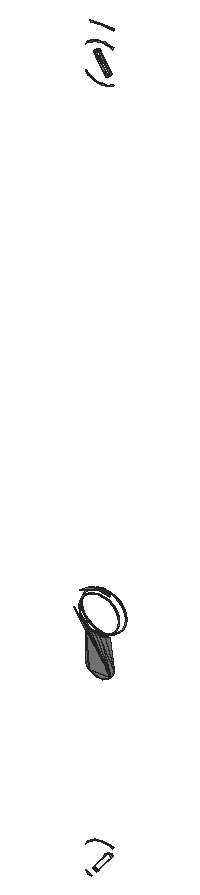
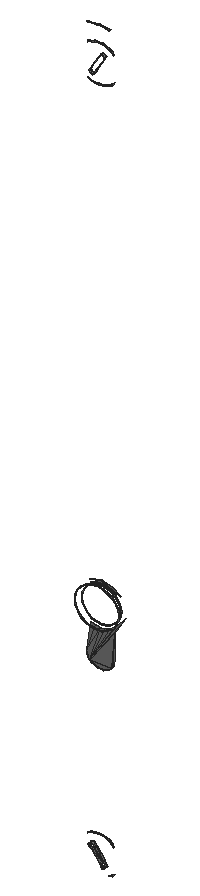
# SketchUp Ruby script. Lengths in inches.
U = 1.inch
M = Sketchup.active_model
def pt(a) = Geom::Point3d.new(a.map { |v| v * U })
def face(e, loops, mat)
  f = e.add_face(loops[0].map { |a| pt(a) })
  loops[1..].each { |l| e.add_face(l.map { |a| pt(a) }).erase! }
  f.material = f.back_material = mat if mat
  f
end
# faces: each face lists its corners as indices into pts; further lists are holes
def faces(e, pts, list, mat = nil) = list.each { |f| face(e, (f[0].is_a?(Array) ? f : [f]).map { |l| l.map { |i| pts[i] } }, mat) }
# xy, xz, yz: faces in a plane at the given z, y or x. An outline is a flat list of corners, or four numbers for a rectangle; further outlines are holes
def ring(l) = l.size == 4 ? [[l[0], l[1]], [l[2], l[1]], [l[2], l[3]], [l[0], l[3]]] : l.each_slice(2).to_a
def flat(e, list, mat, &to3) = list.each { |f| face(e, (f[0].is_a?(Array) ? f : [f]).map { |l| ring(l).map { |u, v| to3.(u, v) } }, mat) }
def xy(e, z, list, mat = nil) = flat(e, list, mat) { |x, y| [x, y, z] }
def xz(e, y, list, mat = nil) = flat(e, list, mat) { |x, z| [x, y, z] }
def yz(e, x, list, mat = nil) = flat(e, list, mat) { |y, z| [x, y, z] }
def lines(e, pts, list) = list.each { |a, b| e.add_line(pt(pts[a]), pt(pts[b])) }
# prism: a flat outline (further loops are holes) pulled along v
def prism(e, loops, v, mat = nil)
  f = face(e, loops, mat); d = Geom::Vector3d.new(v.map { |x| x * U })
  f.pushpull(f.normal.samedirection?(d) ? d.length : -d.length)
end
def box(e, o, s, mat = nil) = prism(e, [[o, [o[0] + s[0], o[1], o[2]], [o[0] + s[0], o[1] + s[1], o[2]], [o[0], o[1] + s[1], o[2]]]], [0, 0, s[2]], mat)
def at(x, y, z, deg = 0) = Geom::Transformation.translation(pt([x, y, z])) * Geom::Transformation.rotation(ORIGIN, Z_AXIS, deg.degrees)
def axes(o, x, y, z) = Geom::Transformation.new([*x, 0, *y, 0, *z, 0, *pt(o).to_a, 1])
def part(name) = M.definitions.add(name)
# library, detail: a bought-in or finely detailed component or shape, given as its bounding box
def library(name, o, s) = part(name).tap { |d| box(d.entities, o, s) }
def detail(e, o, s) = box(e.add_group.entities, o, s)
def put(e, d, t, mat = nil) = e.add_instance(d, t).tap { |i| i.material = mat if mat }
def group(e, t, mat = nil) = e.add_group.tap { |g| g.transformation = t; g.material = mat if mat }.entities
root = M.entities
M.materials.add("Material \#1").color = [140, 140, 140]
xz(root,529.302,[[1590.92,42.491,1590.851,42.499,1590.92,42.5],[1590.92,42.491,1590.92,42.5,1590.987,42.508],[1590.92,42.491,1590.987,42.508,1590.989,42.499],[1590.851,42.499,1590.786,42.523,1590.854,42.508],[1590.851,42.499,1590.854,42.508,1590.92,42.5],
  [1590.989,42.499,1590.987,42.508,1591.049,42.531],[1590.989,42.499,1591.049,42.531,1591.054,42.523],[1590.854,42.508,1590.786,42.523,1590.792,42.531],[1590.786,42.523,1590.731,42.561,1590.792,42.531],[1591.054,42.523,1591.049,42.531,1591.102,42.567],
  [1591.054,42.523,1591.102,42.567,1591.109,42.561],[1590.792,42.531,1590.731,42.561,1590.738,42.567],[1590.731,42.561,1590.689,42.61,1590.738,42.567],[1591.109,42.561,1591.102,42.567,1591.143,42.614],[1591.109,42.561,1591.143,42.614,1591.152,42.61],
  [1590.738,42.567,1590.689,42.61,1590.697,42.614],[1590.689,42.61,1590.662,42.667,1590.697,42.614],[1591.152,42.61,1591.143,42.614,1591.169,42.67],[1591.152,42.61,1591.169,42.67,1591.178,42.667],[1590.697,42.614,1590.662,42.667,1590.672,42.67],
  [1590.662,42.667,1590.653,42.729,1590.672,42.67],[1591.178,42.667,1591.169,42.67,1591.177,42.729],[1591.178,42.667,1591.177,42.729,1591.1875,42.729],[1590.672,42.67,1590.653,42.729,1590.663,42.729],[1590.653,42.729,1590.662,42.791,1590.663,42.729],
  [1590.663,42.729,1590.662,42.791,1590.672,42.788],[1591.177,42.729,1591.169,42.788,1591.1875,42.729],[1591.1875,42.729,1591.169,42.788,1591.178,42.791],[1590.672,42.788,1590.662,42.791,1590.689,42.848],[1590.672,42.788,1590.689,42.848,1590.697,42.843],
  [1591.169,42.788,1591.143,42.843,1591.178,42.791],[1591.178,42.791,1591.143,42.843,1591.152,42.848],[1590.697,42.843,1590.689,42.848,1590.731,42.897],[1590.697,42.843,1590.731,42.897,1590.738,42.891],[1591.143,42.843,1591.102,42.891,1591.152,42.848],
  [1591.152,42.848,1591.102,42.891,1591.109,42.897],[1590.738,42.891,1590.731,42.897,1590.786,42.935],[1590.738,42.891,1590.786,42.935,1590.792,42.927],[1591.102,42.891,1591.049,42.927,1591.109,42.897],[1591.109,42.897,1591.049,42.927,1591.054,42.935],
  [1590.792,42.927,1590.786,42.935,1590.851,42.959],[1590.792,42.927,1590.851,42.959,1590.854,42.95],[1591.049,42.927,1590.987,42.95,1591.054,42.935],[1591.054,42.935,1590.987,42.95,1590.989,42.959],[1590.854,42.95,1590.851,42.959,1590.92,42.967],
  [1590.854,42.95,1590.92,42.967,1590.92,42.958],[1590.987,42.95,1590.92,42.958,1590.989,42.959],[1590.92,42.958,1590.92,42.967,1590.989,42.959]],"Material \#1")
xz(root,529.3125,[[1590.92,41.959,1590.772,42.022,1591.068,42.022],[1590.92,41.959,1590.837,41.976,1590.772,42.022],[1590.92,41.959,1590.877,41.963,1590.837,41.976],[1590.92,41.959,1591.004,41.976,1590.964,41.963],[1590.92,41.959,1591.068,42.022,1591.004,41.976],
  [1590.837,41.976,1590.801,41.996,1590.772,42.022],[1591.004,41.976,1591.068,42.022,1591.039,41.996],[1591.068,42.022,1590.583,42.689,1590.686,42.562],[1591.068,42.022,1590.723,42.477,1590.583,42.689],[1591.068,42.022,1590.686,42.562,1590.733,42.521],
  [1591.068,42.022,1590.726,42.471,1590.723,42.477],[1591.068,42.022,1590.728,42.465,1590.726,42.471],[1591.068,42.022,1590.73,42.459,1590.728,42.465],[1590.772,42.022,1590.73,42.452,1590.73,42.459],[1590.772,42.022,1590.73,42.459,1591.068,42.022],
  [1590.772,42.022,1590.735,42.089,1590.73,42.452],[1591.068,42.022,1590.733,42.521,1590.788,42.489],[1590.772,42.022,1590.749,42.054,1590.735,42.089],[1591.068,42.022,1590.788,42.489,1590.851,42.469],[1591.068,42.022,1590.851,42.469,1590.92,42.462],
  [1591.068,42.022,1590.92,42.462,1591.11,42.128],[1591.068,42.022,1591.105,42.089,1591.091,42.054],[1591.068,42.022,1591.11,42.128,1591.105,42.089],[1590.735,42.089,1590.73,42.128,1590.73,42.452],[1591.11,42.128,1590.92,42.462,1590.989,42.469],
  [1591.11,42.128,1590.989,42.469,1591.052,42.489],[1590.655,42.918,1590.771,43.001,1590.92,43.032],[1590.655,42.918,1590.92,43.032,1590.788,42.969],[1590.788,42.969,1590.92,43.032,1590.851,42.989],[1591.052,42.969,1590.989,42.989,1590.92,43.032],
  [1590.851,42.989,1590.92,43.032,1590.92,42.996],[1590.989,42.989,1590.92,42.996,1590.92,43.032],[1590.771,43.001,1590.842,43.024,1590.92,43.032],[1591.07,43.001,1590.92,43.032,1590.998,43.024]],"Material \#1")
xz(root,529.347,[[1590.781,39.535,1590.733,39.549,1590.743,39.559],[1590.733,39.549,1590.698,39.58,1590.743,39.559],[1590.71,39.905,1590.733,39.945,1590.743,39.934],[1590.743,39.934,1590.733,39.945,1590.774,39.97],[1590.743,39.934,1590.774,39.97,1590.781,39.959],
  [1590.781,39.959,1590.774,39.97,1590.819,39.989],[1590.781,39.959,1590.819,39.989,1590.824,39.977],[1591.059,39.959,1591.016,39.977,1591.067,39.97],[1591.067,39.97,1591.016,39.977,1591.021,39.989],[1590.824,39.977,1590.819,39.989,1590.868,40.001],
  [1590.824,39.977,1590.868,40.001,1590.871,39.988],[1591.016,39.977,1590.969,39.988,1591.021,39.989],[1590.871,39.988,1590.868,40.001,1590.92,40.005],[1590.871,39.988,1590.92,40.005,1590.92,39.992],[1590.969,39.988,1590.92,39.992,1590.972,40.001],
  [1590.969,39.988,1590.972,40.001,1591.021,39.989],[1590.92,39.992,1590.92,40.005,1590.972,40.001],[1590.92,49.013,1590.868,49.017,1590.92,49.027],[1590.92,49.013,1590.92,49.027,1590.969,49.031],[1590.92,49.013,1590.969,49.031,1590.972,49.017],
  [1590.868,49.017,1590.819,49.029,1590.871,49.031],[1590.868,49.017,1590.871,49.031,1590.92,49.027],[1590.972,49.017,1590.969,49.031,1591.016,49.042],[1590.972,49.017,1591.016,49.042,1591.021,49.029],[1590.819,49.029,1590.774,49.049,1590.824,49.042],
  [1590.819,49.029,1590.824,49.042,1590.871,49.031],[1591.021,49.029,1591.016,49.042,1591.059,49.06],[1591.021,49.029,1591.059,49.06,1591.067,49.049],[1590.824,49.042,1590.774,49.049,1590.781,49.06],[1590.774,49.049,1590.733,49.074,1590.781,49.06],
  [1590.781,49.06,1590.733,49.074,1590.743,49.084],[1590.733,49.074,1590.698,49.105,1590.743,49.084],[1590.71,49.43,1590.733,49.47,1590.743,49.459],[1590.743,49.459,1590.733,49.47,1590.774,49.495],[1590.743,49.459,1590.774,49.495,1590.781,49.484],
  [1590.781,49.484,1590.774,49.495,1590.819,49.514],[1590.781,49.484,1590.819,49.514,1590.824,49.502],[1591.059,49.484,1591.016,49.502,1591.067,49.495],[1591.067,49.495,1591.016,49.502,1591.021,49.514],[1590.824,49.502,1590.819,49.514,1590.868,49.526],
  [1590.824,49.502,1590.868,49.526,1590.871,49.513],[1591.016,49.502,1590.969,49.513,1591.021,49.514],[1590.871,49.513,1590.868,49.526,1590.92,49.53],[1590.871,49.513,1590.92,49.53,1590.92,49.517],[1590.969,49.513,1590.92,49.517,1590.972,49.526],
  [1590.969,49.513,1590.972,49.526,1591.021,49.514],[1590.92,49.517,1590.92,49.53,1590.972,49.526],[1590.766,49.713,1590.763,49.726,1590.92,49.739],[1590.766,49.713,1590.92,49.739,1590.92,49.725],[1591.075,49.713,1590.92,49.725,1591.077,49.726],
  [1590.92,49.725,1590.92,49.739,1591.077,49.726]],"Material \#1")
xz(root,529.382,[[1590.92,42.462,1590.843,42.471,1590.92,42.471],[1590.92,42.462,1590.92,42.471,1590.995,42.48],[1590.92,42.462,1590.995,42.48,1590.998,42.471],[1590.843,42.471,1590.77,42.498,1590.845,42.48],[1590.843,42.471,1590.845,42.48,1590.92,42.471],
  [1590.998,42.471,1590.995,42.48,1591.065,42.505],[1590.998,42.471,1591.065,42.505,1591.07,42.498],[1590.845,42.48,1590.77,42.498,1590.775,42.505],[1590.77,42.498,1590.708,42.54,1590.775,42.505],[1591.07,42.498,1591.065,42.505,1591.125,42.546],
  [1591.07,42.498,1591.125,42.546,1591.132,42.54],[1590.775,42.505,1590.708,42.54,1590.715,42.546],[1590.708,42.54,1590.66,42.595,1590.715,42.546],[1591.132,42.54,1591.125,42.546,1591.171,42.6],[1591.132,42.54,1591.171,42.6,1591.18,42.595],
  [1590.715,42.546,1590.66,42.595,1590.669,42.6],[1590.66,42.595,1590.63,42.66,1590.669,42.6],[1591.18,42.595,1591.171,42.6,1591.2,42.662],[1591.18,42.595,1591.2,42.662,1591.21,42.66],[1590.669,42.6,1590.63,42.66,1590.64,42.662],
  [1590.63,42.66,1590.62,42.729,1590.64,42.662],[1591.21,42.66,1591.2,42.662,1591.21,42.729],[1591.21,42.66,1591.21,42.729,1591.22,42.729],[1590.64,42.662,1590.62,42.729,1590.63,42.729],[1590.62,42.729,1590.63,42.798,1590.63,42.729],
  [1590.63,42.729,1590.63,42.798,1590.64,42.796],[1591.21,42.729,1591.2,42.796,1591.22,42.729],[1591.22,42.729,1591.2,42.796,1591.21,42.798],[1590.64,42.796,1590.63,42.798,1590.66,42.862],[1590.64,42.796,1590.66,42.862,1590.669,42.858],
  [1591.2,42.796,1591.171,42.858,1591.21,42.798],[1591.21,42.798,1591.171,42.858,1591.18,42.862],[1590.669,42.858,1590.66,42.862,1590.708,42.918],[1590.669,42.858,1590.708,42.918,1590.715,42.911],[1591.171,42.858,1591.125,42.911,1591.18,42.862],
  [1591.18,42.862,1591.125,42.911,1591.132,42.918],[1590.715,42.911,1590.708,42.918,1590.77,42.96],[1590.715,42.911,1590.77,42.96,1590.775,42.952],[1591.125,42.911,1591.065,42.952,1591.132,42.918],[1591.132,42.918,1591.065,42.952,1591.07,42.96],
  [1590.775,42.952,1590.77,42.96,1590.843,42.987],[1590.775,42.952,1590.843,42.987,1590.845,42.978],[1591.065,42.952,1590.995,42.978,1591.07,42.96],[1591.07,42.96,1590.995,42.978,1590.998,42.987],[1590.845,42.978,1590.843,42.987,1590.92,42.996],
  [1590.845,42.978,1590.92,42.996,1590.92,42.987],[1590.995,42.978,1590.92,42.987,1590.998,42.987],[1590.92,42.987,1590.92,42.996,1590.998,42.987]],"Material \#1")
p = [[1590.82,529.347,39.672],[1590.82,529.374,39.672],[1590.798,529.382,39.644],[1590.798,529.354,39.644],[1590.875,529.374,39.637],[1590.875,529.347,39.637],
  [1590.854,529.354,39.609],[1590.895,529.372,39.662],[1590.895,529.344,39.662],[1590.823,529.382,39.623],[1590.823,529.354,39.623],[1590.854,529.382,39.609],
  [1590.945,529.344,39.831],[1590.945,529.372,39.831],[1590.84,529.372,39.697],[1590.84,529.344,39.697],[1591.001,529.372,39.797],[1591.001,529.344,39.797],
  [1590.965,529.347,39.856],[1590.965,529.374,39.856],[1591.021,529.374,39.822],[1591.02,529.347,39.822],[1591.043,529.382,39.849],[1591.043,529.354,39.849],
  [1591.017,529.382,39.87],[1591.017,529.354,39.87],[1590.987,529.354,39.884],[1590.987,529.382,39.884],[1590.954,529.347,49.159],[1590.954,529.374,49.159],
  [1590.973,529.382,49.13],[1590.973,529.354,49.13],[1591.005,529.382,49.141],[1591.005,529.354,49.141],[1591.032,529.382,49.16],[1591.032,529.354,49.16],
  [1590.845,529.344,49.328],[1590.845,529.372,49.328],[1590.937,529.372,49.186],[1590.937,529.344,49.186],[1590.996,529.344,49.216],[1590.996,529.372,49.216],
  [1590.903,529.372,49.358],[1590.903,529.344,49.358],[1591.013,529.374,49.189],[1591.013,529.347,49.189],[1590.828,529.347,49.354],[1590.828,529.374,49.354],
  [1590.809,529.354,49.384],[1590.886,529.374,49.384],[1590.886,529.347,49.384],[1590.867,529.382,49.414],[1590.867,529.354,49.414],[1590.836,529.382,49.402],
  [1590.836,529.354,49.402],[1590.809,529.382,49.384]]
faces(root,p,[[0,1,2],[2,3,0],[4,5,6],[5,4,7],[7,8,5],[3,2,9],[9,10,3],[10,9,11],
  [11,6,10],[6,11,4],[12,13,14],[14,15,12],[15,14,1],[1,0,15],[8,7,16],[16,17,8],
  [18,19,13],[13,12,18],[17,16,20],[20,21,17],[21,20,22],[22,23,21],[23,22,24],[24,25,23],
  [19,18,26],[25,24,27],[27,26,25],[26,27,19],[28,29,30],[30,31,28],[31,30,32],[32,33,31],
  [33,32,34],[34,35,33],[36,37,38],[38,39,36],[39,38,29],[29,28,39],[40,41,42],[42,43,40],
  [44,45,35],[45,44,41],[41,40,45],[35,34,44],[46,47,37],[37,36,46],[47,46,48],[43,42,49],
  [49,50,43],[50,49,51],[51,52,50],[52,51,53],[53,54,52],[54,53,55],[55,48,54],[48,55,47]],"Material \#1")
